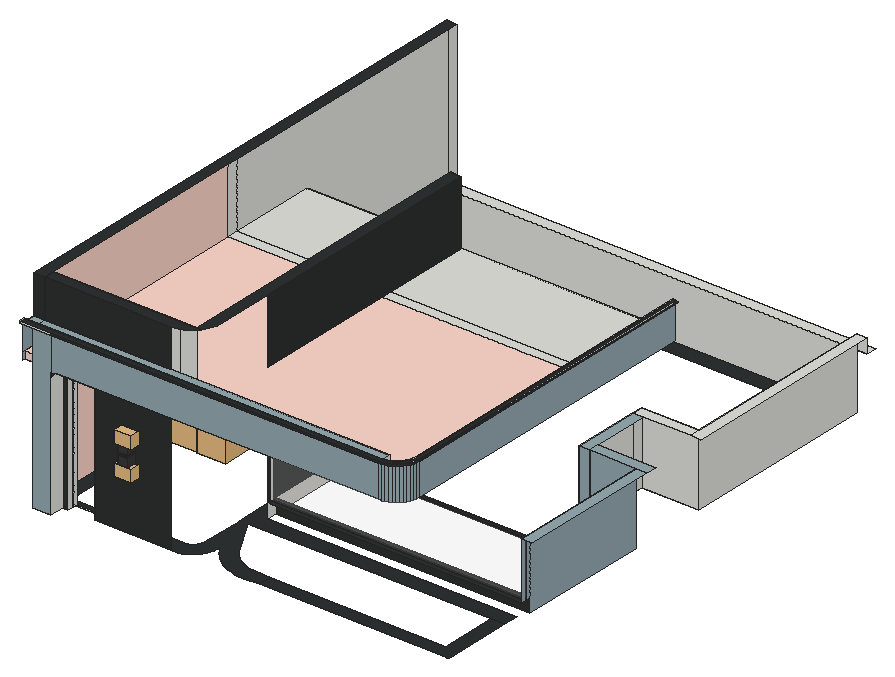
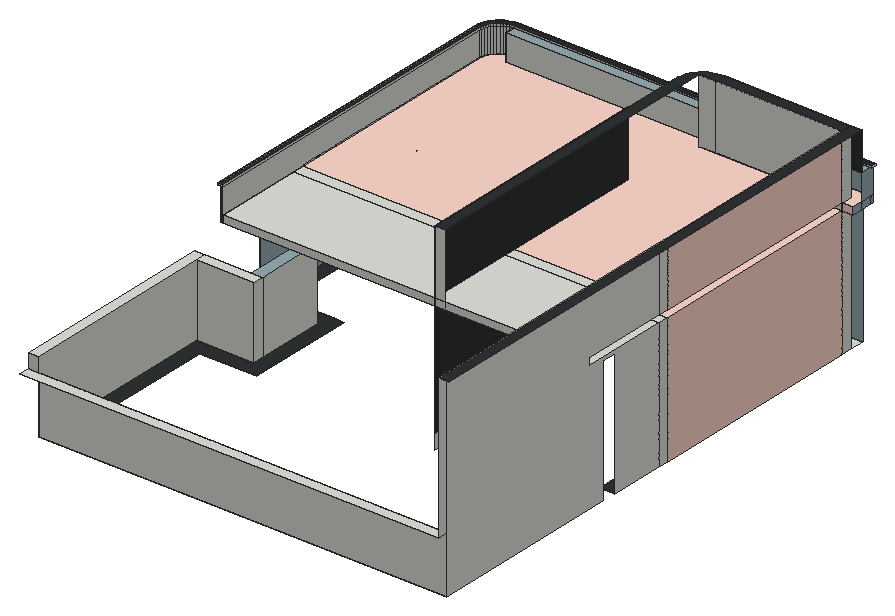
# SketchUp Ruby script. Lengths in inches.
U = 1.inch
M = Sketchup.active_model
def pt(a) = Geom::Point3d.new(a.map { |v| v * U })
def face(e, loops, mat)
  f = e.add_face(loops[0].map { |a| pt(a) })
  loops[1..].each { |l| e.add_face(l.map { |a| pt(a) }).erase! }
  f.material = f.back_material = mat if mat
  f
end
# faces: each face lists its corners as indices into pts; further lists are holes
def faces(e, pts, list, mat = nil) = list.each { |f| face(e, (f[0].is_a?(Array) ? f : [f]).map { |l| l.map { |i| pts[i] } }, mat) }
# xy, xz, yz: faces in a plane at the given z, y or x. An outline is a flat list of corners, or four numbers for a rectangle; further outlines are holes
def ring(l) = l.size == 4 ? [[l[0], l[1]], [l[2], l[1]], [l[2], l[3]], [l[0], l[3]]] : l.each_slice(2).to_a
def flat(e, list, mat, &to3) = list.each { |f| face(e, (f[0].is_a?(Array) ? f : [f]).map { |l| ring(l).map { |u, v| to3.(u, v) } }, mat) }
def xy(e, z, list, mat = nil) = flat(e, list, mat) { |x, y| [x, y, z] }
def xz(e, y, list, mat = nil) = flat(e, list, mat) { |x, z| [x, y, z] }
def yz(e, x, list, mat = nil) = flat(e, list, mat) { |y, z| [x, y, z] }
def lines(e, pts, list) = list.each { |a, b| e.add_line(pt(pts[a]), pt(pts[b])) }
# prism: a flat outline (further loops are holes) pulled along v
def prism(e, loops, v, mat = nil)
  f = face(e, loops, mat); d = Geom::Vector3d.new(v.map { |x| x * U })
  f.pushpull(f.normal.samedirection?(d) ? d.length : -d.length)
end
def box(e, o, s, mat = nil) = prism(e, [[o, [o[0] + s[0], o[1], o[2]], [o[0] + s[0], o[1] + s[1], o[2]], [o[0], o[1] + s[1], o[2]]]], [0, 0, s[2]], mat)
def at(x, y, z, deg = 0) = Geom::Transformation.translation(pt([x, y, z])) * Geom::Transformation.rotation(ORIGIN, Z_AXIS, deg.degrees)
def axes(o, x, y, z) = Geom::Transformation.new([*x, 0, *y, 0, *z, 0, *pt(o).to_a, 1])
def part(name) = M.definitions.add(name)
# library, detail: a bought-in or finely detailed component or shape, given as its bounding box
def library(name, o, s) = part(name).tap { |d| box(d.entities, o, s) }
def detail(e, o, s) = box(e.add_group.entities, o, s)
def put(e, d, t, mat = nil) = e.add_instance(d, t).tap { |i| i.material = mat if mat }
def group(e, t, mat = nil) = e.add_group.tap { |g| g.transformation = t; g.material = mat if mat }.entities
root = M.entities
M.materials.add("11.free-metal-textures").color = [58, 58, 58]
M.materials.add("Emissive").color = [234, 228, 175]
M.materials.add("Generic").color = [150, 171, 178]
M.materials.add("Generic\#1").color = [47, 50, 50]
M.materials.add("Glass Thin Clear 001").color = [252, 250, 250]
M.materials["Glass Thin Clear 001"].alpha = 0.1
M.materials.add("[0111_SlateGray]").color = [112, 128, 144]
M.materials.add("[0117_GhostWhite]").color = [248, 248, 255]
M.materials.add("[Color B01]").color = [255, 216, 204]
M.materials.add("images").color = [124, 124, 124]
c1 = library("Omni Light\#1",[-12,-12,-12],[24,24,24])
c2 = library("Spot Light",[-7.3,-7.3,-9.9375],[14.6,14.6,9.9375])
c3 = part("Group0\#1")
p = [[-17.97,0.98,0],[-6.48,-16.79,0],[0,0,38],[13.97,-11.35,0],[15.11,9.78,0],[-4.625,17.4,0]]
faces(c3.entities,p,[[0,1,2],[1,3,2],[3,4,2],[5,0,2],[4,5,2]])
c4 = part("wall light")
g1 = group(c4.entities,at(188.14,62.59,-1.03))
xy(g1,0.24,[[[0,0,7.875,7.875],[0.49,0.49,7.38,7.38]]],"images")
xy(g1,1.03,[[[0.49,0.49,7.38,7.38],[0.73,0.73,7.14,7.14]]],"[0111_SlateGray]")
xy(g1,2.21,[[0.73,0.73,7.14,7.14]],"[0117_GhostWhite]")
xy(g1,5.75,[[2.36,13.78,5.51,14.17]],"images")
xy(g1,6.74,[[3.35,7.875,4.52,13.78]],"images")
xy(g1,7.72,[[0,0,7.875,0,7.875,7.875,7.38,7.875,7.38,0.49,0.49,0.49,0.49,7.875,0,7.875],[0.49,7.38,7.38,7.875]])
xy(g1,8.5,[[3.35,9.63,4.52,12.02]])
xy(g1,8.51,[[0,0,0,7.875,0.49,7.875,0.49,0.49,7.38,0.49,7.38,7.875,7.875,7.875,7.875,0]])
xy(g1,9.29,[[0,0,7.875,0,7.875,7.875,7.38,7.875,7.38,0.49,0.49,0.49,0.49,7.875,0,7.875]])
xy(g1,9.3,[[3.35,9.63,4.52,12.02]])
xy(g1,10.08,[[0,0,7.875,0,7.875,7.875,7.38,7.875,7.38,0.49,0,0.49],[0,0.49,0.49,7.875],[0.49,7.38,7.38,7.875]])
xy(g1,11.06,[[3.35,7.875,4.52,13.78]],"images")
xy(g1,12.05,[[2.36,13.78,5.51,14.17]],"images")
xy(g1,15.59,[[0.73,0.73,7.14,7.14]],"[0117_GhostWhite]")
xy(g1,16.77,[[[0.49,0.49,7.38,7.38],[0.73,0.73,7.14,7.14]]],"[0111_SlateGray]")
xy(g1,17.5625,[[[0,0,7.875,7.875],[0.49,0.49,7.38,7.38]]],"images")
xz(g1,0,[[0,0.24,7.875,7.72],[0,8.51,7.875,9.29],[0,10.08,7.875,17.5625]],"11.free-metal-textures")
xz(g1,0.49,[[0.49,8.51,7.38,8.9],[0.49,8.9,7.38,9.29]])
xz(g1,0.49,[[0.49,0.24,7.38,1.03],[0.49,16.77,7.38,17.5625]],"[0111_SlateGray]")
xz(g1,0.49,[[0.49,7.72,7.38,8.51],[0.49,9.29,7.38,10.08]],"[0117_GhostWhite]")
xz(g1,0.73,[[0.73,1.03,7.14,2.21],[0.73,2.21,7.14,15.59],[0.73,15.59,7.14,16.77]],"[0111_SlateGray]")
xz(g1,7.14,[[0.73,1.03,7.14,2.21],[0.73,2.21,7.14,15.59],[0.73,15.59,7.14,16.77]],"[0111_SlateGray]")
xz(g1,7.38,[[0.49,0.24,7.38,1.03],[0.49,16.77,7.38,17.5625]],"[0111_SlateGray]")
xz(g1,7.875,[[3.35,6.74,4.52,7.72],[3.35,7.72,3.9375,10.08],[3.9375,7.72,4.52,10.08],[3.35,10.08,4.52,11.06]])
xz(g1,7.875,[[0,0.24,0,7.72,3.35,7.72,3.35,6.74,4.52,6.74,4.52,7.72,7.875,7.72,7.875,0.24],[0.49,7.72,0.49,8.51,0,8.51,0,9.29,0.49,9.29,0.49,10.08,3.35,10.08,3.35,7.72],[4.52,7.72,4.52,10.08,7.38,10.08,7.38,9.29,7.875,9.29,7.875,8.51,7.38,8.51,7.38,7.72],[0,10.08,0,17.5625,7.875,17.5625,7.875,10.08,4.52,10.08,4.52,11.06,3.35,11.06,3.35,10.08]],"11.free-metal-textures")
xz(g1,9.63,[[3.35,8.5,4.52,9.3]])
xz(g1,12.02,[[3.35,8.5,4.52,9.3]])
xz(g1,13.78,[[2.36,5.75,4.52,5.75,4.52,6.74,3.35,6.74,3.35,11.06,4.52,11.06,4.52,5.75,5.51,5.75,5.51,12.05,2.36,12.05]],"images")
xz(g1,14.17,[[2.36,5.75,5.51,12.05]])
yz(g1,0,[[0,0.24,7.875,7.72],[0,8.51,7.875,9.29],[0,10.08,7.875,17.5625]],"11.free-metal-textures")
yz(g1,0.49,[[0.49,8.51,7.38,8.9]])
yz(g1,0.49,[[0.49,0.24,7.38,1.03],[0.49,16.77,7.38,17.5625]],"[0111_SlateGray]")
yz(g1,0.49,[[0.49,7.72,7.875,8.51],[0.49,9.29,7.875,10.08]],"[0117_GhostWhite]")
yz(g1,0.73,[[0.73,1.03,7.14,2.21],[0.73,2.21,7.14,15.59],[0.73,15.59,7.14,16.77]],"[0111_SlateGray]")
yz(g1,2.36,[[13.78,5.75,14.17,12.05]],"images")
yz(g1,3.35,[[[7.875,6.74,13.78,11.06],[9.63,8.5,12.02,9.3]]],"images")
yz(g1,4.52,[[[7.875,6.74,13.78,11.06],[9.63,8.5,12.02,9.3]]],"images")
yz(g1,5.51,[[13.78,5.75,14.17,12.05]],"images")
yz(g1,7.14,[[0.73,1.03,7.14,2.21],[0.73,2.21,7.14,15.59],[0.73,15.59,7.14,16.77]],"[0111_SlateGray]")
yz(g1,7.38,[[0.49,8.51,7.38,8.9]])
yz(g1,7.38,[[0.49,0.24,7.38,1.03],[0.49,16.77,7.38,17.5625]],"[0111_SlateGray]")
yz(g1,7.38,[[0.49,7.72,7.875,8.51],[0.49,9.29,7.875,10.08]],"[0117_GhostWhite]")
yz(g1,7.875,[[0,0.24,7.875,7.72],[0,8.51,7.875,9.29],[0,10.08,7.875,17.5625]],"11.free-metal-textures")
p = [[7.38,7.38,8.9],[0.49,7.38,8.9],[4.52,7.875,6.54],[4.52,7.875,6.74],[4.52,13.78,5.5625],[4.52,13.78,5.75]]
lines(g1,p,[[0,1],[2,3],[4,5]])
put(g1,c3,axes([3.74,4.28,0],[0.1617,0,0],[0,0.1617,0],[0,0,0.1617]))
put(g1,c3,axes([4.15,3.625,18],[-0.1617,0,0],[0,0.1617,0],[0,0,-0.1617]))
c5 = library("Tlon Light 650 Ceiling 152 007",[-12.8,-12.8,-3.78],[25.6,25.6,3.58])
xy(root,390,[[10.218,29.933,25.218,42.0625],[29.81,49.75,51.935,51.0625]])
xy(root,390,[[10.218,42.0625,29.81,42.0625,29.81,51.0625,51.935,51.0625,51.935,42.0625,120.213,42.0625,121.268,42.29,122.311,42.565,123.34,42.889,124.353,43.259,125.348,43.676,126.323,44.138,127.276,44.644,128.204,45.194,129.105,45.786,129.979,46.419,130.822,47.092,131.634,47.803,132.412,48.55,133.154,49.332,133.86,50.148,134.528,50.996,135.155,51.873,135.742,52.778,136.286,53.71,136.787,54.665,137.244,55.643,137.654,56.64,138.019,57.655,138.336,58.686,138.605,59.731,138.826,60.787,138.998,61.852,139.121,62.924,139.194,64,139.218,65.078,141.135,61.721,143.351,58.552,145.848,55.6,148.603,52.887,151.595,50.438,154.798,48.272,158.186,46.408,161.729,44.861,165.4,43.645,169.165,42.768,172.996,42.239,176.858,42.0625,189.581,42.785,189.581,54.216,174.159,54.922,171.482,55.292,168.851,55.904,166.286,56.754,163.81,57.835,161.442,59.138,159.204,60.652,157.113,62.363,155.1875,64.259,153.443,66.322,151.894,68.536,133.159,101.34,348.495,101.34,348.495,114.0625,139.218,114.0625,139.218,135.785,126.495,135.785,126.495,101.34,127.285,101.34,126.481,64.571,126.447,64.08,126.391,63.591,126.313,63.105,126.212,62.623,126.089,62.147,125.945,61.676,125.778,61.213,125.591,60.758,125.383,60.312,125.154,59.876,124.906,59.451,124.638,59.038,124.352,58.638,124.047,58.251,123.725,57.879,123.386,57.522,123.031,57.181,122.661,56.856,122.276,56.549,121.878,56.261,121.466,55.99,121.043,55.74,120.608,55.508,120.163,55.298,119.709,55.107,119.247,54.938,118.777,54.791,118.756,54.785,22.94,54.785,22.94,289.296,10.218,289.296],[189.581,42.785,345.414,42.785,345.816,42.811,346.211,42.89,346.593,43.02,346.954,43.198,347.289,43.422,347.593,43.6875,347.858,43.991,348.082,44.326,348.26,44.687,348.39,45.069,348.469,45.464,348.495,45.866,348.495,101.34,337.064,101.34,337.064,54.216,189.581,54.216],[139.218,123.0625,352.218,123.0625,352.218,234.034,313.218,234.034,313.218,234.0625,304.218,234.0625,304.218,300.0625,352.218,300.0625,352.218,465.0625,10.218,465.0625,10.218,302.163,22.94,302.163,22.94,452.34,339.495,452.34,339.495,312.785,291.495,312.785,291.495,221.34,300.495,221.34,300.495,221.311,339.495,221.311,339.495,135.785,139.218,135.785]],"Generic\#1")
xy(root,402,[[139.218,114.0625,352.218,117.694],[139.218,119.431,352.218,123.0625]],"Generic\#1")
xy(root,438,[[10.218,465.0625,361.218,474.0625]])
xy(root,449.179,[[138.536,117.012,352.899,120.113]],"Generic\#1")
xy(root,450,[[304.218,291.0625,352.218,300.0625],[352.218,291.0625,361.218,465.0625]])
xy(root,450,[[352.218,114.0625,361.218,234.034],[313.218,234.034,361.218,243.0625],[304.218,234.0625,313.218,291.0625]],"Generic")
xy(root,495.3125,[[10.218,289.296,130.218,302.163]])
xy(root,495.654,[[29.81,42.0625,51.935,46.096],[29.81,46.096,51.935,47.721],[29.81,47.721,51.935,51.0625]])
xy(root,498,[[30.424,29.933,299.703,32.125],[299.703,29.933,299.703,32.125,301.9,32.269,304.058,32.698,306.143,33.406,308.117,34.379,309.947,35.602,311.602,37.053,313.053,38.708,314.276,40.538,315.249,42.512,315.957,44.597,316.386,46.755,316.53,48.952,316.53,317.038,318.718,317.038,318.718,48.952,318.5,46.49,317.973,44.076,317.145,41.748,316.03,39.543,314.644,37.497,313.012,35.642,311.157,34.009,309.111,32.623,306.907,31.507,304.579,30.679,302.165,30.151],[10.218,234.0625,316.53,243.0625],[10.218,243.0625,316.53,317.038]])
xy(root,498,[[[1.218,32.125,1.218,51.0625,10.218,51.0625,10.218,234.0625,316.53,234.0625,316.53,48.952,316.386,46.755,315.957,44.597,315.249,42.512,314.276,40.538,313.053,38.708,311.602,37.053,309.947,35.602,308.117,34.379,306.143,33.406,304.058,32.698,301.9,32.269,299.703,32.125],[21.894,43.802,299.703,43.802,300.375,43.846,301.036,43.977,301.674,44.194,302.278,44.492,302.839,44.866,303.345,45.31,303.789,45.817,304.164,46.377,304.461,46.981,304.678,47.619,304.809,48.28,304.854,48.952,304.854,222.386,21.894,222.386]],[[24.408,46.315,24.408,219.872,302.34,219.872,302.34,48.952,302.317,48.608,302.25,48.269,302.139,47.943,301.987,47.634,301.795,47.347,301.568,47.088,301.308,46.86,301.022,46.669,300.712,46.516,300.386,46.405,300.047,46.338,299.703,46.315],[227.204,97.562,232.443,97.856,237.622,98.696,242.685,100.073,247.576,101.972,252.241,104.372,256.631,107.246,260.696,110.563,264.392,114.287,267.678,118.377,270.519,122.788,272.884,127.471,274.745,132.377,276.084,137.45,276.885,142.635,277.14,147.875,276.846,153.114,276.006,158.293,274.629,163.355,272.73,168.246,270.33,172.912,267.456,177.302,264.139,181.367,260.415,185.0625,256.325,188.349,251.914,191.19,247.231,193.554,242.325,195.416,237.252,196.755,232.067,197.556,226.827,197.811,221.588,197.517,216.409,196.676,211.347,195.299,206.456,193.401,201.79,191.001,197.4,188.127,193.335,184.81,189.639,181.086,186.353,176.996,183.512,172.585,181.148,167.901,179.286,162.996,177.947,157.923,177.146,152.738,176.891,147.498,177.185,142.259,178.026,137.08,179.403,132.017,181.301,127.126,183.701,122.461,186.575,118.071,189.892,114.006,193.616,110.31,197.706,107.024,202.117,104.183,206.801,101.818,211.706,99.957,216.779,98.618,221.964,97.817]]],"[Color B01]")
xy(root,500.0625,[[[21.894,43.802,21.894,222.386,304.854,222.386,304.854,48.952,304.809,48.28,304.678,47.619,304.461,46.981,304.164,46.377,303.789,45.817,303.345,45.31,302.839,44.866,302.278,44.492,301.674,44.194,301.036,43.977,300.375,43.846,299.703,43.802],[24.408,46.315,299.703,46.315,300.047,46.338,300.386,46.405,300.712,46.516,301.022,46.669,301.308,46.86,301.568,47.088,301.795,47.347,301.987,47.634,302.139,47.943,302.25,48.269,302.317,48.608,302.34,48.952,302.34,219.872,24.408,219.872]]],"Emissive")
xy(root,502,[[227.204,97.562,221.964,97.817,216.779,98.618,211.706,99.957,206.801,101.818,202.117,104.183,197.706,107.024,193.616,110.31,189.892,114.006,186.575,118.071,183.701,122.461,181.301,127.126,179.403,132.017,178.026,137.08,177.185,142.259,176.891,147.498,177.146,152.738,177.947,157.923,179.286,162.996,181.148,167.901,183.512,172.585,186.353,176.996,189.639,181.086,193.335,184.81,197.4,188.127,201.79,191.001,206.456,193.401,211.347,195.299,216.409,196.676,221.588,197.517,226.827,197.811,232.067,197.556,237.252,196.755,242.325,195.416,247.231,193.554,251.914,191.19,256.325,188.349,260.415,185.0625,264.139,181.367,267.456,177.302,270.33,172.912,272.73,168.246,274.629,163.355,276.006,158.293,276.846,153.114,277.14,147.875,276.885,142.635,276.084,137.45,274.745,132.377,272.884,127.471,270.519,122.788,267.678,118.377,264.392,114.287,260.696,110.563,256.631,107.246,252.241,104.372,247.576,101.972,242.685,100.073,237.622,98.696,232.443,97.856]],"[Color B01]")
xy(root,504.044,[[25.218,32.125,299.703,42.0625],[10.218,234.0625,316.53,243.0625],[10.218,243.0625,316.53,317.038]])
xy(root,504.044,[[1.218,32.125,25.218,32.125,25.218,42.0625,299.703,42.0625,299.703,32.125,301.9,32.269,304.058,32.698,306.143,33.406,308.117,34.379,309.947,35.602,311.602,37.053,313.053,38.708,314.276,40.538,315.249,42.512,315.957,44.597,316.386,46.755,316.53,48.952,316.53,234.0625,10.218,234.0625,10.218,51.0625,1.218,51.0625]],"[Color B01]")
xy(root,525.75,[[0,28.716,0,33.343,299.663,33.343,299.703,33.345,301.74,33.479,303.743,33.877,305.676,34.533,307.507,35.436,309.204,36.57,310.739,37.916,312.085,39.451,313.219,41.149,314.122,42.979,314.778,44.913,315.176,46.915,315.3125,48.992,315.3125,318.256,319.935,318.256,319.935,48.898,319.706,46.306,319.146,43.741,318.267,41.267,317.081,38.924,315.609,36.75,313.874,34.78,311.904,33.044,309.73,31.572,307.388,30.386,304.914,29.506,302.349,28.945,299.757,28.716]])
xy(root,525.75,[[1.218,33.343,10.218,42.0625],[10.218,33.343,299.663,33.343,299.703,33.345,299.703,42.0625,10.218,42.0625]],"Generic")
xy(root,527.165,[[0,28.716,299.757,28.716,302.349,28.945,304.914,29.506,307.388,30.386,309.73,31.572,311.904,33.044,313.874,34.78,315.609,36.75,317.081,38.924,318.267,41.267,319.146,43.741,319.706,46.306,319.935,48.898,319.935,318.256,315.3125,318.256,315.3125,48.992,315.176,46.915,314.778,44.913,314.122,42.979,313.219,41.149,312.085,39.451,310.739,37.916,309.204,36.57,307.507,35.436,305.676,34.533,303.743,33.877,301.74,33.479,299.663,33.343,0,33.343]],"Generic\#1")
xy(root,558,[[1.218,42.0625,10.218,474.0625],[10.218,42.0625,116.202,42.0625,119.206,42.259,122.159,42.847,125.009,43.814,127.71,45.146,130.213,46.819,132.476,48.804,134.457,51.0625,10.218,51.0625],[130.218,51.0625,134.457,51.0625,134.461,51.067,136.134,53.57,137.466,56.271,138.433,59.121,139.021,62.074,139.218,65.078,139.218,317.038,130.218,317.038]],"Generic\#1")
xz(root,28.716,[[0,525.75,10.218,527.165],[10.218,525.75,25.218,527.165]])
xz(root,28.716,[[25.218,525.75,299.757,527.165]],"Generic\#1")
xz(root,29.494,[[3.849,525.75,299.789,527.165]])
xz(root,29.933,[[10.218,390,25.218,525.75],[25.218,493.469,25.22,493.496,25.38,494.228,25.642,494.93,26.002,495.588,26.452,496.188,26.983,496.718,27.583,497.167,28.241,497.526,28.944,497.787,29.676,497.947,30.424,498,299.703,498,299.703,525.75,25.218,525.75]],"Generic")
xz(root,32.125,[[25.218,492,25.218,493.469,25.165,492.748],[25.218,493.469,25.218,498,30.424,498,29.676,497.947,28.944,497.787,28.241,497.526,27.583,497.167,26.983,496.718,26.452,496.188,26.002,495.588,25.642,494.93,25.38,494.228,25.22,493.496],[25.218,504.044,299.703,525.75]])
xz(root,32.125,[[1.218,498,25.218,504.044],[25.218,498,299.703,504.044]],"[Color B01]")
xz(root,32.564,[[3.849,525.75,299.587,527.165]])
xz(root,33.343,[[0,525.75,10.218,527.165],[10.218,525.75,25.218,527.165],[25.218,525.75,299.663,527.165]])
xz(root,42.0625,[[10.218,390,10.218,525.75,116.202,525.75,116.202,504.044,25.218,504.044,25.218,390],[116.202,504.044,299.703,525.75]])
xz(root,42.0625,[[25.218,390,29.81,390,29.81,495.654,51.935,495.654,51.935,390,116.202,390,116.202,504.044,25.218,504.044],[1.218,525.75,10.218,558],[10.218,525.75,116.202,558]],"Generic\#1")
xz(root,43.802,[[30.424,498,299.703,500.0625]],"Emissive")
xz(root,43.802,[[21.894,498,25.218,500.0625],[25.218,498,30.424,500.0625]],"[Color B01]")
xz(root,46.315,[[30.424,498,299.703,500.0625]],"Emissive")
xz(root,46.315,[[24.408,498,25.218,500.0625],[25.218,498,30.424,500.0625]],"[Color B01]")
xz(root,51.0625,[[10.218,498,116.202,504.044],[116.202,498,130.218,504.044],[10.218,504.044,116.202,558],[116.202,504.044,130.218,558]])
xz(root,51.0625,[[1.218,498,130.218,504.044],[130.218,498,134.457,504.044]],"[Color B01]")
xz(root,117.012,[[352.218,448.5625,352.899,449.179]])
xz(root,117.012,[[138.536,448.5625,352.218,449.179]],"Generic\#1")
xz(root,117.048,[[141.601,448.5625,349.834,449.179]])
xz(root,117.694,[[139.218,402,352.218,448.5625]],"Glass Thin Clear 001")
xz(root,119.431,[[139.218,402,352.218,448.5625]],"Glass Thin Clear 001")
xz(root,120.077,[[141.601,448.5625,349.834,449.179]])
xz(root,120.113,[[138.536,448.5625,352.899,449.179]])
xz(root,123.0625,[[139.218,390,352.218,402]],"Generic\#1")
xz(root,219.872,[[24.408,498,302.34,500.0625]],"[Color B01]")
xz(root,222.386,[[21.894,498,304.854,500.0625]],"Emissive")
xz(root,234.034,[[313.218,390,352.218,450]],"Generic")
xz(root,234.0625,[[304.218,390,313.218,450]],"Generic")
xz(root,300.0625,[[304.218,390,352.218,450]])
xz(root,317.038,[[10.218,498,130.218,504.044],[130.218,498,139.218,504.044],[139.218,498,316.53,504.044],[316.53,498,318.718,525.75],[130.218,504.044,139.218,558]])
xz(root,318.256,[[315.3125,525.75,319.935,527.165]])
xz(root,465.0625,[[10.218,390,352.218,438],[352.218,438,361.218,450]])
yz(root,0,[[28.716,525.75,33.343,527.165]])
yz(root,1.218,[[29.933,498,32.125,504.044],[32.125,498,42.0625,504.044],[42.0625,498,51.0625,504.044],[29.933,504.044,42.0625,525.75]],"Generic")
yz(root,10.218,[[42.0625,390,51.0625,558],[234.0625,390,243.0625,498],[243.0625,390,289.296,390,289.296,495.3125,302.163,495.3125,302.163,390,465.0625,390,465.0625,558,243.0625,558,243.0625,504.044,317.038,504.044,317.038,498,243.0625,498],[465.0625,438,474.0625,558],[234.0625,504.044,243.0625,558]])
yz(root,10.218,[[51.0625,390,234.0625,498],[51.0625,504.044,234.0625,558]],"[Color B01]")
yz(root,21.894,[[43.802,498,51.0625,500.0625],[51.0625,498,222.386,500.0625]],"[Color B01]")
yz(root,24.408,[[46.315,498,51.0625,500.0625],[51.0625,498,219.872,500.0625]],"[Color B01]")
yz(root,25.218,[[29.933,390,42.0625,390,42.0625,504.044,32.125,504.044,32.125,493.469,29.933,493.469],[29.933,493.469,32.125,496.375]])
yz(root,29.81,[[42.0625,390,46.096,495.654],[46.096,390,47.721,495.654],[47.721,390,51.0625,495.654]])
yz(root,51.935,[[42.0625,390,46.096,495.654],[46.096,390,47.721,495.654],[47.721,390,51.0625,495.654]])
yz(root,138.536,[[117.012,448.5625,120.113,449.179]])
yz(root,139.218,[[114.0625,390,123.0625,390,123.0625,402,119.431,402,119.431,448.5625,117.694,448.5625,117.694,402,114.0625,402],[123.0625,390,317.038,402]])
yz(root,139.218,[[114.0625,402,117.694,402,117.694,448.5625,119.431,448.5625,119.431,402,317.038,402,317.038,558,114.0625,558]],"Generic\#1")
yz(root,299.703,[[32.125,504.044,42.0625,525.75]])
yz(root,302.34,[[48.952,498,219.872,500.0625]],"Emissive")
yz(root,304.218,[[234.0625,390,291.0625,450],[291.0625,390,300.0625,450]])
yz(root,304.854,[[48.952,498,222.386,500.0625]],"Emissive")
yz(root,313.218,[[234.034,390,234.0625,450]])
yz(root,315.3125,[[48.992,525.75,318.256,527.165]])
yz(root,316.087,[[49.068,525.75,314.407,527.165]])
yz(root,316.53,[[48.952,498,234.0625,504.044],[234.0625,498,243.0625,504.044],[243.0625,498,317.038,504.044],[48.952,504.044,317.038,525.75]])
yz(root,318.718,[[48.952,498,317.038,525.75]],"Generic")
yz(root,319.161,[[48.866,525.75,314.407,527.165]])
yz(root,319.935,[[48.898,525.75,318.256,527.165]],"Generic\#1")
yz(root,352.218,[[300.0625,390,465.0625,450]])
yz(root,352.218,[[123.0625,390,234.034,450],[114.0625,402,114.0625,450,123.0625,450,123.0625,402,119.431,402,119.431,448.5625,120.077,448.5625,120.077,449.179,117.012,449.179,117.012,448.5625,117.694,448.5625,117.694,402]],"Generic")
yz(root,352.899,[[117.012,448.5625,120.113,449.179]])
p = [[25.218,32.125,493.469],[25.22,32.125,493.496],[25.22,29.933,493.496],[25.218,29.933,493.469],[25.38,32.125,494.228],[25.38,29.933,494.228],
  [25.642,32.125,494.93],[25.642,29.933,494.93],[26.002,32.125,495.588],[26.002,29.933,495.588],[26.452,32.125,496.188],[26.452,29.933,496.188],
  [26.983,32.125,496.718],[26.983,29.933,496.718],[27.583,32.125,497.167],[27.583,29.933,497.167],[28.241,32.125,497.526],[28.241,29.933,497.526],
  [28.944,32.125,497.787],[28.944,29.933,497.787],[29.676,32.125,497.947],[29.676,29.933,497.947],[30.424,32.125,498],[30.424,29.933,498],
  [299.703,29.933,498],[302.165,30.151,498],[302.165,30.151,525.75],[299.703,29.933,525.75],[304.579,30.679,498],[304.579,30.679,525.75],
  [306.907,31.507,498],[306.907,31.507,525.75],[309.111,32.623,498],[309.111,32.623,525.75],[299.703,32.125,504.044],[301.9,32.269,504.044],
  [301.9,32.269,498],[299.703,32.125,498],[304.058,32.698,504.044],[304.058,32.698,498],[311.157,34.009,498],[311.157,34.009,525.75],
  [306.143,33.406,504.044],[306.143,33.406,498],[308.117,34.379,504.044],[308.117,34.379,498],[313.012,35.642,498],[313.012,35.642,525.75],
  [309.947,35.602,504.044],[309.947,35.602,498],[311.602,37.053,504.044],[311.602,37.053,498],[314.644,37.497,498],[314.644,37.497,525.75],
  [313.053,38.708,504.044],[313.053,38.708,498],[316.03,39.543,498],[316.03,39.543,525.75],[314.276,40.538,504.044],[314.276,40.538,498],
  [317.145,41.748,498],[317.145,41.748,525.75],[315.249,42.512,504.044],[315.249,42.512,498],[317.973,44.076,498],[317.973,44.076,525.75],
  [315.957,44.597,504.044],[315.957,44.597,498],[300.375,43.846,498],[299.703,43.802,498],[299.703,43.802,500.0625],[300.375,43.846,500.0625],
  [301.036,43.977,498],[301.036,43.977,500.0625],[301.674,44.194,498],[301.674,44.194,500.0625],[318.5,46.49,498],[318.5,46.49,525.75],
  [302.278,44.492,498],[302.278,44.492,500.0625],[302.839,44.866,498],[302.839,44.866,500.0625],[316.386,46.755,504.044],[316.386,46.755,498],
  [303.345,45.31,498],[303.345,45.31,500.0625],[303.789,45.817,498],[303.789,45.817,500.0625],[304.164,46.377,498],[304.164,46.377,500.0625],
  [299.703,46.315,498],[300.047,46.338,498],[300.047,46.338,500.0625],[299.703,46.315,500.0625],[300.386,46.405,498],[300.386,46.405,500.0625],
  [300.712,46.516,498],[300.712,46.516,500.0625],[304.461,46.981,498],[304.461,46.981,500.0625],[301.022,46.669,498],[301.022,46.669,500.0625],
  [318.718,48.952,498],[318.718,48.952,525.75],[301.308,46.86,498],[301.308,46.86,500.0625],[316.53,48.952,504.044],[316.53,48.952,498],
  [301.568,47.088,498],[301.568,47.088,500.0625],[304.678,47.619,498],[304.678,47.619,500.0625],[301.795,47.347,498],[301.795,47.347,500.0625],
  [301.987,47.634,498],[301.987,47.634,500.0625],[302.139,47.943,498],[302.139,47.943,500.0625],[304.809,48.28,498],[304.809,48.28,500.0625],
  [302.25,48.269,498],[302.25,48.269,500.0625],[302.317,48.608,498],[302.317,48.608,500.0625],[304.854,48.952,498],[304.854,48.952,500.0625],
  [302.34,48.952,498],[302.34,48.952,500.0625],[227.204,97.562,498],[221.964,97.817,498],[221.964,97.817,502],[227.204,97.562,502],
  [232.443,97.856,498],[232.443,97.856,502],[216.779,98.618,498],[216.779,98.618,502],[237.622,98.696,498],[237.622,98.696,502],
  [211.706,99.957,498],[211.706,99.957,502],[242.685,100.073,498],[242.685,100.073,502],[206.801,101.818,498],[206.801,101.818,502],
  [247.576,101.972,498],[247.576,101.972,502],[202.117,104.183,498],[202.117,104.183,502],[252.241,104.372,498],[252.241,104.372,502],
  [197.706,107.024,498],[197.706,107.024,502],[256.631,107.246,498],[256.631,107.246,502],[193.616,110.31,498],[193.616,110.31,502],
  [260.696,110.563,498],[260.696,110.563,502],[189.892,114.006,498],[189.892,114.006,502],[264.392,114.287,498],[264.392,114.287,502],
  [186.575,118.071,498],[186.575,118.071,502],[267.678,118.377,498],[267.678,118.377,502],[183.701,122.461,498],[183.701,122.461,502],
  [270.519,122.788,498],[270.519,122.788,502],[181.301,127.126,498],[181.301,127.126,502],[272.884,127.471,498],[272.884,127.471,502],
  [179.403,132.017,498],[179.403,132.017,502],[274.745,132.377,498],[274.745,132.377,502],[178.026,137.08,498],[178.026,137.08,502],
  [276.084,137.45,498],[276.084,137.45,502],[177.185,142.259,498],[177.185,142.259,502],[276.885,142.635,498],[276.885,142.635,502],
  [176.891,147.498,498],[176.891,147.498,502],[277.14,147.875,498],[277.14,147.875,502],[177.146,152.738,498],[177.146,152.738,502],
  [276.846,153.114,498],[276.846,153.114,502],[177.947,157.923,498],[177.947,157.923,502],[276.006,158.293,498],[276.006,158.293,502],
  [179.286,162.996,498],[179.286,162.996,502],[274.629,163.355,498],[274.629,163.355,502],[181.148,167.901,498],[181.148,167.901,502],
  [272.73,168.246,498],[272.73,168.246,502],[183.512,172.585,498],[183.512,172.585,502],[270.33,172.912,498],[270.33,172.912,502],
  [186.353,176.996,498],[186.353,176.996,502],[267.456,177.302,498],[267.456,177.302,502],[189.639,181.086,498],[189.639,181.086,502],
  [264.139,181.367,498],[264.139,181.367,502],[193.335,184.81,498],[193.335,184.81,502],[260.415,185.0625,498],[260.415,185.0625,502],
  [197.4,188.127,498],[197.4,188.127,502],[256.325,188.349,498],[256.325,188.349,502],[201.79,191.001,498],[201.79,191.001,502],
  [251.914,191.19,498],[251.914,191.19,502],[206.456,193.401,498],[206.456,193.401,502],[247.231,193.554,498],[247.231,193.554,502],
  [211.347,195.299,498],[211.347,195.299,502],[242.325,195.416,498],[242.325,195.416,502],[216.409,196.676,498],[216.409,196.676,502],
  [237.252,196.755,498],[237.252,196.755,502],[221.588,197.517,498],[221.588,197.517,502],[232.067,197.556,498],[232.067,197.556,502],
  [226.827,197.811,498],[226.827,197.811,502],[301.9,32.269,525.75],[299.703,32.125,525.75],[304.058,32.698,525.75],[306.143,33.406,525.75],
  [308.117,34.379,525.75],[309.947,35.602,525.75],[311.602,37.053,525.75],[313.053,38.708,525.75],[314.276,40.538,525.75],[315.249,42.512,525.75],
  [315.957,44.597,525.75],[316.386,46.755,525.75],[316.53,48.952,525.75],[302.349,28.945,525.75],[302.349,28.945,527.165],[299.757,28.716,527.165],
  [299.757,28.716,525.75],[304.914,29.506,525.75],[304.914,29.506,527.165],[299.789,29.494,527.165],[299.789,29.494,525.75],[302.244,29.655,525.75],
  [302.244,29.655,527.165],[307.388,30.386,525.75],[307.388,30.386,527.165],[304.73,30.15,525.75],[304.741,30.152,525.75],[304.741,30.152,527.165],
  [304.73,30.15,527.165],[307.152,30.97,525.75],[307.152,30.97,527.165],[309.73,31.572,525.75],[309.73,31.572,527.165],[309.435,32.096,525.75],
  [309.435,32.096,527.165],[309.425,32.091,527.165],[311.904,33.044,525.75],[311.904,33.044,527.165],[311.552,33.51,525.75],[311.552,33.51,527.165],
  [301.766,32.757,527.165],[301.766,32.757,525.75],[299.703,32.575,525.75],[299.689,32.573,525.75],[299.587,32.564,525.75],[299.587,32.564,527.165],
  [299.689,32.573,527.165],[303.854,33.213,527.165],[303.854,33.213,525.75],[301.833,32.772,525.75],[313.874,34.78,525.75],[313.874,34.78,527.165],
  [305.867,33.93,527.165],[305.867,33.93,525.75],[303.915,33.235,527.165],[299.663,33.343,525.75],[299.663,33.343,527.165],[301.74,33.479,527.165],
  [301.74,33.479,525.75],[299.703,33.345,525.75],[303.743,33.877,527.165],[303.743,33.877,525.75],[313.466,35.189,525.75],[313.466,35.189,527.165],
  [305.676,34.533,527.165],[305.676,34.533,525.75],[307.774,34.895,527.165],[307.774,34.895,525.75],[307.507,35.436,527.165],[307.507,35.436,525.75],
  [315.609,36.75,525.75],[315.609,36.75,527.165],[309.544,36.094,527.165],[309.544,36.094,525.75],[315.145,37.103,525.75],[315.145,37.103,527.165],
  [309.204,36.57,527.165],[309.204,36.57,525.75],[311.147,37.506,527.165],[311.147,37.506,525.75],[310.739,37.916,527.165],[310.739,37.916,525.75],
  [317.081,38.924,525.75],[317.081,38.924,527.165],[315.148,37.108,525.75],[316.559,39.22,525.75],[316.559,39.22,527.165],[315.148,37.108,527.165],
  [312.559,39.11,527.165],[312.559,39.11,525.75],[311.148,37.507,525.75],[311.148,37.507,527.165],[312.547,39.096,527.165],[312.085,39.451,527.165],
  [312.085,39.451,525.75],[318.267,41.267,525.75],[318.267,41.267,527.165],[313.758,40.88,527.165],[313.758,40.88,525.75],[313.737,40.849,525.75],
  [316.563,39.229,525.75],[317.685,41.504,525.75],[317.685,41.504,527.165],[316.563,39.229,527.165],[313.219,41.149,527.165],[313.219,41.149,525.75],
  [314.722,42.787,527.165],[314.722,42.787,525.75],[314.699,42.74,525.75],[314.699,42.74,527.165],[314.122,42.979,527.165],[314.122,42.979,525.75],
  [319.146,43.741,525.75],[319.146,43.741,527.165],[317.689,41.515,525.75],[318.503,43.914,525.75],[318.503,43.914,527.165],[315.438,44.8,527.165],
  [315.438,44.8,525.75],[315.417,44.741,525.75],[314.778,44.913,527.165],[314.778,44.913,525.75],[319.706,46.306,525.75],[319.706,46.306,527.165],
  [319,46.411,525.75],[319,46.411,527.165],[318.505,43.924,527.165],[315.894,46.888,527.165],[315.894,46.888,525.75],[315.88,46.822,525.75],
  [315.88,46.822,527.165],[315.176,46.915,527.165],[315.176,46.915,525.75],[319.935,48.898,525.75],[319.935,48.898,527.165],[319.161,48.866,525.75],
  [319.161,48.866,527.165],[319,46.414,527.165],[315.3125,48.992,527.165],[315.3125,48.992,525.75],[316.087,49.068,527.165],[316.087,49.068,525.75],
  [316.078,48.967,525.75],[316.078,48.967,527.165]]
faces(root,p,[[0,1,2,3],[1,4,5,2],[4,6,7,5],[6,8,9,7],[8,10,11,9],[10,12,13,11],[12,14,15,13],[14,16,17,15],
  [16,18,19,17],[18,20,21,19],[20,22,23,21],[248,35,34,249],[250,38,35,248],[251,42,38,250],[252,44,42,251],[253,48,44,252],
  [254,50,48,253],[255,54,50,254],[256,58,54,255],[257,62,58,256],[258,66,62,257],[259,82,66,258],[260,106,82,259],[267,268,269,270],
  [270,269,273,274,275,276],[275,274,277,278],[278,277,281,282,283],[282,281,286,287],[288,289,290,291,292,293,294],[295,296,297,289,288],[300,301,296,295,302],[303,304,305,306,307],
  [306,305,308,309],[287,286,310,311],[309,308,312,313],[314,315,301,300],[313,312,316,317],[320,321,315,314],[311,310,322,323],[317,316,324,325],
  [326,327,321,320],[325,324,328,329],[323,322,332,333,334,335],[336,337,338,327,326,339,340],[329,328,341,342],[345,346,347,337,336],[334,333,348,349,350,351],[342,341,352,353],
  [354,355,356,346,345,357],[353,352,358,359],[350,349,362,363,364],[365,366,367,355,354],[359,358,368,369],[364,363,372,373,374],[375,376,377,366,365,378],[369,368,379,380],
  [373,372,383,384,385],[380,379,386,387],[388,389,390,376,375,391]])
faces(root,p,[[24,25,26,27],[25,28,29,26],[28,30,31,29],[30,32,33,31],[32,40,41,33],[40,46,47,41],[46,52,53,47],[52,56,57,53],
  [56,60,61,57],[60,64,65,61],[64,76,77,65],[76,102,103,77]],"Generic")
faces(root,p,[[34,35,36,37],[35,38,39,36],[38,42,43,39],[42,44,45,43],[44,48,49,45],[48,50,51,49],[50,54,55,51],[54,58,59,55],
  [58,62,63,59],[62,66,67,63],[66,82,83,67],[82,106,107,83]],"[Color B01]")
faces(root,p,[[68,69,70,71],[72,68,71,73],[74,72,73,75],[78,74,75,79],[80,78,79,81],[84,80,81,85],[86,84,85,87],[88,86,87,89],
  [90,91,92,93],[91,94,95,92],[94,96,97,95],[98,88,89,99],[96,100,101,97],[100,104,105,101],[104,108,109,105],[110,98,99,111],
  [108,112,113,109],[112,114,115,113],[114,116,117,115],[118,110,111,119],[116,120,121,117],[120,122,123,121],[124,118,119,125],[122,126,127,123],
  [128,129,130,131],[132,128,131,133],[129,134,135,130],[136,132,133,137],[134,138,139,135],[140,136,137,141],[138,142,143,139],[144,140,141,145],
  [142,146,147,143],[148,144,145,149],[146,150,151,147],[152,148,149,153],[150,154,155,151],[156,152,153,157],[154,158,159,155],[160,156,157,161],
  [158,162,163,159],[164,160,161,165],[162,166,167,163],[168,164,165,169],[166,170,171,167],[172,168,169,173],[170,174,175,171],[176,172,173,177],
  [174,178,179,175],[180,176,177,181],[178,182,183,179],[184,180,181,185],[182,186,187,183],[188,184,185,189],[186,190,191,187],[192,188,189,193],
  [190,194,195,191],[196,192,193,197],[194,198,199,195],[200,196,197,201],[198,202,203,199],[204,200,201,205],[202,206,207,203],[208,204,205,209],
  [206,210,211,207],[212,208,209,213],[210,214,215,211],[216,212,213,217],[214,218,219,215],[220,216,217,221],[218,222,223,219],[224,220,221,225],
  [222,226,227,223],[228,224,225,229],[226,230,231,227],[232,228,229,233],[230,234,235,231],[236,232,233,237],[234,238,239,235],[240,236,237,241],
  [238,242,243,239],[244,240,241,245],[242,246,247,243],[246,244,245,247]],"Emissive")
faces(root,p,[[261,262,263,264],[265,266,262,261],[271,272,266,265],[279,280,272,271],[284,285,280,279],[298,299,285,284],[318,319,299,298],[330,331,319,318],
  [343,344,331,330],[360,361,344,343],[370,371,361,360],[381,382,371,370]],"Generic\#1")
put(root,c1,at(63.63,131.15,427.5))
put(root,c1,at(24.45,131.15,427.5))
put(root,c1,at(87.95,131.15,427.5))
put(root,c2,at(81.74,41,444.6))
put(root,c4,at(-110.42,-27.91,444.71))
put(root,c2,axes([81.74,41,459.77],[1,0,0],[0,1,0],[0,0,-1]))
put(root,c5,axes([275.42,56.54,498.34],[0.17,0,0],[0,0.17,0],[0,0,0.17]))
put(root,c5,axes([218.54,56.54,498.34],[0.17,0,0],[0,0.17,0],[0,0,0.17]))
put(root,c5,axes([161.67,56.54,498.34],[0.17,0,0],[0,0.17,0],[0,0,0.17]))
put(root,c5,axes([275.42,210.17,498.34],[0.17,0,0],[0,0.17,0],[0,0,0.17]))
put(root,c5,axes([161.67,210.17,498.34],[0.17,0,0],[0,0.17,0],[0,0,0.17]))
put(root,c5,axes([218.54,210.17,498.34],[0.17,0,0],[0,0.17,0],[0,0,0.17]))
put(root,c5,axes([288.42,148.23,498.34],[0.17,0,0],[0,0.17,0],[0,0,0.17]))
put(root,c5,axes([161.67,148.23,498.34],[0.17,0,0],[0,0.17,0],[0,0,0.17]))
